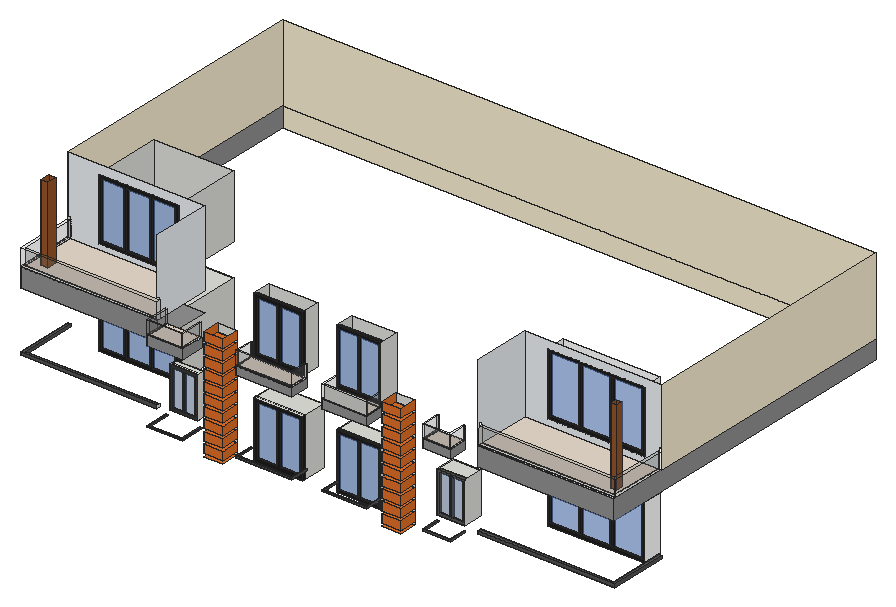
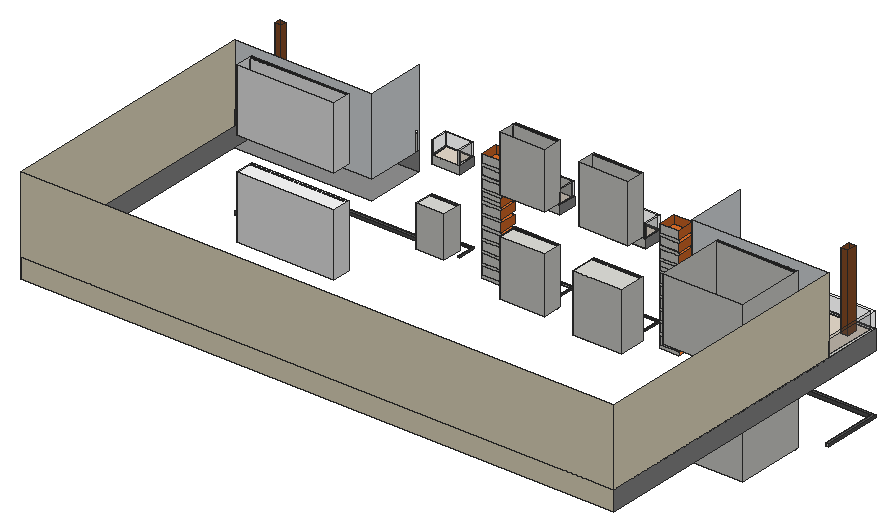
# SketchUp Ruby script. Lengths in inches.
U = 1.inch
M = Sketchup.active_model
def pt(a) = Geom::Point3d.new(a.map { |v| v * U })
def face(e, loops, mat)
  f = e.add_face(loops[0].map { |a| pt(a) })
  loops[1..].each { |l| e.add_face(l.map { |a| pt(a) }).erase! }
  f.material = f.back_material = mat if mat
  f
end
# faces: each face lists its corners as indices into pts; further lists are holes
def faces(e, pts, list, mat = nil) = list.each { |f| face(e, (f[0].is_a?(Array) ? f : [f]).map { |l| l.map { |i| pts[i] } }, mat) }
# xy, xz, yz: faces in a plane at the given z, y or x. An outline is a flat list of corners, or four numbers for a rectangle; further outlines are holes
def ring(l) = l.size == 4 ? [[l[0], l[1]], [l[2], l[1]], [l[2], l[3]], [l[0], l[3]]] : l.each_slice(2).to_a
def flat(e, list, mat, &to3) = list.each { |f| face(e, (f[0].is_a?(Array) ? f : [f]).map { |l| ring(l).map { |u, v| to3.(u, v) } }, mat) }
def xy(e, z, list, mat = nil) = flat(e, list, mat) { |x, y| [x, y, z] }
def xz(e, y, list, mat = nil) = flat(e, list, mat) { |x, z| [x, y, z] }
def yz(e, x, list, mat = nil) = flat(e, list, mat) { |y, z| [x, y, z] }
def lines(e, pts, list) = list.each { |a, b| e.add_line(pt(pts[a]), pt(pts[b])) }
# prism: a flat outline (further loops are holes) pulled along v
def prism(e, loops, v, mat = nil)
  f = face(e, loops, mat); d = Geom::Vector3d.new(v.map { |x| x * U })
  f.pushpull(f.normal.samedirection?(d) ? d.length : -d.length)
end
def box(e, o, s, mat = nil) = prism(e, [[o, [o[0] + s[0], o[1], o[2]], [o[0] + s[0], o[1] + s[1], o[2]], [o[0], o[1] + s[1], o[2]]]], [0, 0, s[2]], mat)
def at(x, y, z, deg = 0) = Geom::Transformation.translation(pt([x, y, z])) * Geom::Transformation.rotation(ORIGIN, Z_AXIS, deg.degrees)
def axes(o, x, y, z) = Geom::Transformation.new([*x, 0, *y, 0, *z, 0, *pt(o).to_a, 1])
def part(name) = M.definitions.add(name)
# library, detail: a bought-in or finely detailed component or shape, given as its bounding box
def library(name, o, s) = part(name).tap { |d| box(d.entities, o, s) }
def detail(e, o, s) = box(e.add_group.entities, o, s)
def put(e, d, t, mat = nil) = e.add_instance(d, t).tap { |i| i.material = mat if mat }
def group(e, t, mat = nil) = e.add_group.tap { |g| g.transformation = t; g.material = mat if mat }.entities
root = M.entities
M.materials.add("Generic").color = [146, 146, 146]
M.materials.add("Generic\#3").color = [226, 112, 41]
M.materials.add("Generic\#4").color = [237, 241, 244]
M.materials.add("Generic\#5").color = [249, 239, 211]
M.materials.add("Generic\#7").color = [232, 220, 205]
M.materials.add("[Color M00]").color = [255, 255, 255]
M.materials.add("[Color M06]").color = [86, 86, 86]
M.materials.add("[Color M07]").color = [58, 58, 58]
M.materials.add("[Color M08]").color = [30, 30, 30]
M.materials.add("[Translucent Glass Blue]").color = [98, 147, 234]
M.materials["[Translucent Glass Blue]"].alpha = 0.27
M.materials.add("[Translucent Glass Blue]1").color = [100, 149, 237]
M.materials["[Translucent Glass Blue]1"].alpha = 0.5
M.materials.add("[Translucent Glass Gray]").color = [119, 119, 119]
M.materials["[Translucent Glass Gray]"].alpha = 0.16
M.materials.add("[Wood Cherry Original]").color = [150, 85, 41]
M.materials.add("[Wood Cherry Original]1").color = [152, 86, 42]
c1 = part("Group\#10")
xy(c1.entities,0,[[0,0,98.1875,6]],"[Color M08]")
xy(c1.entities,5.79,[[5.79,0,46.2,3],[51.99,0,92.4,3]],"[Color M08]")
xy(c1.entities,117.02,[[5.79,0,46.2,3],[51.99,0,92.4,3]],"[Color M08]")
xy(c1.entities,122.8125,[[0,0,98.1875,6]],"[Color M08]")
xz(c1.entities,0,[[[0,0,98.1875,122.8125],[5.79,5.79,46.2,117.02],[51.99,5.79,92.4,117.02]]],"[Color M08]")
xz(c1.entities,3,[[5.79,5.79,46.2,117.02],[51.99,5.79,92.4,117.02]],"[Translucent Glass Blue]1")
xz(c1.entities,6,[[0,0,98.1875,122.8125]])
yz(c1.entities,0,[[0,0,6,122.8125]],"[Color M08]")
yz(c1.entities,5.79,[[0,5.79,3,117.02]],"[Color M08]")
yz(c1.entities,46.2,[[0,5.79,3,117.02]],"[Color M08]")
yz(c1.entities,51.99,[[0,5.79,3,117.02]],"[Color M08]")
yz(c1.entities,92.4,[[0,5.79,3,117.02]],"[Color M08]")
yz(c1.entities,98.1875,[[0,0,6,122.8125]],"[Color M08]")
c2 = part("Group\#11")
xy(c2.entities,0,[[0,0,175.8125,6]],"[Color M08]")
xy(c2.entities,7.33,[[7.33,0,56.16,3],[63.49,0,112.32,3],[119.65,0,168.48,3]],"[Color M08]")
xy(c2.entities,131.1,[[7.33,0,56.16,3],[63.49,0,112.32,3],[119.65,0,168.48,3]],"[Color M08]")
xy(c2.entities,138.4375,[[0,0,175.8125,6]],"[Color M08]")
xz(c2.entities,0,[[[0,0,175.8125,0,175.8125,131.1,168.48,131.1,168.48,7.33,119.65,7.33,119.65,131.1,175.8125,131.1,175.8125,138.4375,0,138.4375],[7.33,7.33,56.16,131.1],[63.49,7.33,112.32,131.1]]],"[Color M08]")
xz(c2.entities,3,[[7.33,7.33,56.16,131.1],[63.49,7.33,112.32,131.1],[119.65,7.33,168.48,131.1]],"[Translucent Glass Blue]1")
xz(c2.entities,6,[[0,0,175.8125,138.4375]])
yz(c2.entities,0,[[0,0,6,138.4375]],"[Color M08]")
yz(c2.entities,7.33,[[0,7.33,3,131.1]],"[Color M08]")
yz(c2.entities,56.16,[[0,7.33,3,131.1]],"[Color M08]")
yz(c2.entities,63.49,[[0,7.33,3,131.1]],"[Color M08]")
yz(c2.entities,112.32,[[0,7.33,3,131.1]],"[Color M08]")
yz(c2.entities,119.65,[[0,7.33,3,131.1]],"[Color M08]")
yz(c2.entities,168.48,[[0,7.33,3,131.1]],"[Color M08]")
yz(c2.entities,175.8125,[[0,0,6,138.4375]],"[Color M08]")
c3 = part("Group\#12")
xy(c3.entities,0,[[0,0,212.5625,7]],"[Color M08]")
xy(c3.entities,6.29,[[6.29,0,68.76,4],[75.05,0,137.52,4],[143.8,0,206.27,4]],"[Color M08]")
xy(c3.entities,131.21,[[6.29,0,68.76,4],[75.05,0,137.52,4],[143.8,0,206.27,4]],"[Color M08]")
xy(c3.entities,137.5,[[0,0,212.5625,7]],"[Color M08]")
xz(c3.entities,0,[[0,0,212.5625,6.29],[0,6.29,6.29,131.21],[68.76,6.29,75.05,131.21],[137.52,6.29,143.8,131.21],[206.27,6.29,212.5625,131.21],
  [0,131.21,212.5625,137.5]],"[Color M08]")
xz(c3.entities,4,[[6.29,6.29,68.76,131.21],[75.05,6.29,137.52,131.21],[143.8,6.29,206.27,131.21]],"[Translucent Glass Blue]1")
xz(c3.entities,7,[[0,0,212.5625,137.5]],"[Color M00]")
yz(c3.entities,0,[[0,0,7,137.5]],"[Color M08]")
yz(c3.entities,6.29,[[0,6.29,4,131.21]],"[Color M08]")
yz(c3.entities,68.76,[[0,6.29,4,131.21]],"[Color M08]")
yz(c3.entities,75.05,[[0,6.29,4,131.21]],"[Color M08]")
yz(c3.entities,137.52,[[0,6.29,4,131.21]],"[Color M08]")
yz(c3.entities,143.8,[[0,6.29,4,131.21]],"[Color M08]")
yz(c3.entities,206.27,[[0,6.29,4,131.21]],"[Color M08]")
yz(c3.entities,212.5625,[[0,0,7,137.5]],"[Color M08]")
c4 = part("Group\#1")
xy(c4.entities,0,[[0,0,60.75,6]],"[Color M07]")
xy(c4.entities,5.51,[[5.51,0,27.62,3],[33.13,0,55.24,3]],"[Color M07]")
xy(c4.entities,84.62,[[5.51,0,27.62,3],[33.13,0,55.24,3]])
xy(c4.entities,90.125,[[0,0,60.75,6]],"[Color M07]")
xz(c4.entities,0,[[[0,0,60.75,90.125],[5.51,5.51,27.62,84.62],[33.13,5.51,55.24,84.62]]],"[Color M07]")
xz(c4.entities,3,[[5.51,5.51,27.62,84.62],[33.13,5.51,55.24,84.62]],"[Translucent Glass Blue]")
xz(c4.entities,6,[[0,0,60.75,90.125]])
yz(c4.entities,0,[[0,0,6,90.125]],"[Color M07]")
yz(c4.entities,5.51,[[0,5.51,3,84.62]],"[Color M07]")
yz(c4.entities,27.62,[[0,5.51,3,84.62]],"[Color M07]")
yz(c4.entities,33.13,[[0,5.51,3,84.62]],"[Color M07]")
yz(c4.entities,55.24,[[0,5.51,3,84.62]],"[Color M07]")
yz(c4.entities,60.75,[[0,0,6,90.125]],"[Color M07]")
c5 = part("Group\#2")
xy(c5.entities,0,[[0,0,60.75,6]],"[Color M06]")
xy(c5.entities,4.875,[[4.875,0,27.9375,3],[32.8125,0,55.875,3]],"[Color M06]")
xy(c5.entities,85.25,[[4.875,0,27.9375,3],[32.8125,0,55.875,3]],"[Color M06]")
xy(c5.entities,90.125,[[0,0,60.75,6]],"[Color M06]")
xz(c5.entities,0,[[[0,0,60.75,90.125],[4.875,4.875,27.9375,85.25],[32.8125,4.875,55.875,85.25]]],"[Color M06]")
xz(c5.entities,3,[[4.875,4.875,27.9375,85.25],[32.8125,4.875,55.875,85.25]],"[Translucent Glass Blue]")
xz(c5.entities,6,[[0,0,60.75,90.125]])
yz(c5.entities,0,[[0,0,6,90.125]],"[Color M06]")
yz(c5.entities,4.875,[[0,4.875,3,85.25]],"[Color M06]")
yz(c5.entities,27.9375,[[0,4.875,3,85.25]],"[Color M06]")
yz(c5.entities,32.8125,[[0,4.875,3,85.25]],"[Color M06]")
yz(c5.entities,55.875,[[0,4.875,3,85.25]],"[Color M06]")
yz(c5.entities,60.75,[[0,0,6,90.125]],"[Color M06]")
xy(root,849.87,[[643.375,273.75,685.0625,313.625],[1034.5,273.75,1076.1875,313.625]],"Generic\#3")
xy(root,850.52,[[722.84,313.625,830.21,370.9375]])
xy(root,853.59,[[903.71,313.625,1001.9,356.375]])
xy(root,853.63,[[276.39,444.3125,452.2,595.9375]])
xy(root,856.37,[[643.375,273.75,685.0625,313.625],[1034.5,273.75,1076.1875,313.625]],"Generic\#3")
xy(root,856.82,[[1262.61,444.3125,1475.18,486.125]],"[Color M00]")
xy(root,873,[[529.46,261.625,529.46,313.625,532.46,313.625,532.46,264.625,604.09,264.625,604.09,313.625,607.09,313.625,607.09,261.625],[714.9,273.75,838.15,276.75],[903.71,273.75,906.71,313.625],[906.71,273.75,1001.9,276.75],[1125.09,273.75,1185.84,276.75],
  [714.9,276.75,717.9,313.625],[835.15,276.75,838.15,313.625],[998.9,276.75,1001.9,313.625],[1125.09,276.75,1128.09,313.625],[1182.84,276.75,1185.84,313.625]])
xy(root,874.37,[[643.375,273.75,685.0625,313.625],[1034.5,273.75,1076.1875,313.625]],"Generic\#3")
xy(root,875.75,[[529.46,261.625,607.09,261.625,607.09,313.625,604.09,313.625,604.09,264.625,532.46,264.625,532.46,313.625,529.46,313.625]],"[Color M06]")
xy(root,876,[[714.9,273.75,838.15,273.75,838.15,313.625,835.15,313.625,835.15,276.75,717.9,276.75,717.9,313.625,714.9,313.625],[903.71,273.75,1001.9,273.75,1001.9,313.625,998.9,313.625,998.9,276.75,906.71,276.75,906.71,313.625,903.71,313.625],[1125.09,273.75,1185.84,273.75,1185.84,313.625,1182.84,313.625,1182.84,276.75,1128.09,276.75,1128.09,313.625,1125.09,313.625]],"[Color M06]")
xy(root,879,[[209.5,313.625,209.5,444.3125,216.5,444.3125,216.5,320.625,509.5,320.625,509.5,313.625],[1213,316.0625,1213,323.0625,1506,323.0625,1506,444.3125,1513,444.3125,1513,316.0625]])
xy(root,880.87,[[643.375,273.75,685.0625,313.625],[1034.5,273.75,1076.1875,313.625]],"Generic\#3")
xy(root,885.4375,[[1213,316.0625,1513,316.0625,1513,444.3125,1506,444.3125,1506,323.0625,1213,323.0625]],"[Color M06]")
xy(root,886,[[209.5,313.625,509.5,313.625,509.5,320.625,216.5,320.625,216.5,444.3125,209.5,444.3125]],"[Color M06]")
xy(root,886.27,[[537.9,313.625,598.65,331.25]])
xy(root,887.24,[[1125.09,313.625,1185.84,356.375]])
xy(root,898.87,[[643.375,273.75,685.0625,313.625],[1034.5,273.75,1076.1875,313.625]],"Generic\#3")
xy(root,905.37,[[643.375,273.75,685.0625,313.625],[1034.5,273.75,1076.1875,313.625]],"Generic\#3")
xy(root,923.37,[[643.375,273.75,685.0625,313.625],[1034.5,273.75,1076.1875,313.625]],"Generic\#3")
xy(root,929.87,[[643.375,273.75,685.0625,313.625],[1034.5,273.75,1076.1875,313.625]],"Generic\#3")
xy(root,947.87,[[643.375,273.75,685.0625,313.625],[1034.5,273.75,1076.1875,313.625]],"Generic\#3")
xy(root,954.37,[[643.375,273.75,685.0625,313.625],[1034.5,273.75,1076.1875,313.625]],"Generic\#3")
xy(root,972.37,[[643.375,273.75,685.0625,313.625],[1034.5,273.75,1076.1875,313.625]],"Generic\#3")
xy(root,976.4,[[537.9,313.625,598.65,331.25],[722.84,313.625,830.21,370.9375],[903.71,313.625,1001.9,356.375]])
xy(root,977.36,[[1125.09,313.625,1185.84,356.375]])
xy(root,978.87,[[643.375,273.75,685.0625,313.625],[1034.5,273.75,1076.1875,313.625]],"Generic\#3")
xy(root,992.07,[[276.39,444.3125,452.2,595.9375]])
xy(root,994.32,[[1262.61,444.3125,1475.18,486.125]],"[Color M00]")
xy(root,996.87,[[643.375,273.75,685.0625,313.625],[1034.5,273.75,1076.1875,313.625]],"Generic\#3")
xy(root,1003.37,[[643.375,273.75,685.0625,313.625],[1034.5,273.75,1076.1875,313.625]],"Generic\#3")
xy(root,1011,[[[209.5,313.625,509.5,444.3125],[234.12,340.02,249.74,361.77]],[[1213,313.625,1513,444.3125],[1483.76,340.63,1497.19,353.98]]],"Generic")
xy(root,1021.37,[[643.375,273.75,685.0625,313.625],[1034.5,273.75,1076.1875,313.625]],"Generic\#3")
xy(root,1027.87,[[643.375,273.75,685.0625,313.625],[1034.5,273.75,1076.1875,313.625]],"Generic\#3")
xy(root,1032.375,[[529.46,261.625,607.09,313.625]],"Generic")
xy(root,1035.3125,[[714.9,273.75,838.15,313.625],[903.71,273.75,1001.9,313.625],[1125.09,273.75,1185.84,313.625]],"Generic")
xy(root,1045.87,[[643.375,273.75,685.0625,313.625],[1034.5,273.75,1076.1875,313.625]],"Generic\#3")
xy(root,1052.37,[[643.375,273.75,685.0625,313.625],[1034.5,273.75,1076.1875,313.625]],"Generic\#3")
xy(root,1053.75,[[529.46,261.625,529.46,313.625,532.46,313.625,532.46,264.625,604.09,264.625,604.09,313.625,607.09,313.625,607.09,261.625],[714.9,273.75,838.15,276.75],[903.71,273.75,1001.9,276.75],[1125.09,273.75,1185.84,276.75],[714.9,276.75,717.9,313.625],
  [835.15,276.75,838.15,313.625],[903.71,276.75,906.71,313.625],[998.9,276.75,1001.9,313.625],[1125.09,276.75,1128.09,313.625],[1182.84,276.75,1185.84,313.625],
  [209.5,313.625,509.5,320.625],[1213,313.625,1513,318.25],[1213,318.25,1213,325.0625,1506,325.0625,1506,444.3125,1513,444.3125,1513,318.25],[209.5,320.625,216.5,444.3125],[234.12,340.02,249.74,361.77],
  [1483.76,340.63,1497.19,353.98]])
xy(root,1053.75,[[532.46,264.625,604.09,313.625],[717.9,276.75,835.15,313.625],[906.71,276.75,998.9,313.625],[1128.09,276.75,1182.84,313.625],[[216.5,320.625,509.5,444.3125],[234.12,340.02,249.74,361.77]],
  [[1213,325.0625,1506,444.3125],[1483.76,340.63,1497.19,353.98]]],"Generic\#7")
xy(root,1056.17,[[722.84,313.625,830.21,354]])
xy(root,1059.34,[[903.71,313.625,1001.9,356.375]])
xy(root,1063.63,[[276.39,444.3125,452.2,595.9375]])
xy(root,1067.01,[[1262.61,444.3125,1475.18,486.125]],"[Color M00]")
xy(root,1070.37,[[643.375,273.75,685.0625,313.625],[1034.5,273.75,1076.1875,313.625]],"Generic\#3")
xy(root,1076.87,[[643.375,273.75,685.0625,313.625],[1034.5,273.75,1076.1875,313.625]],"Generic\#3")
xz(root,261.625,[[529.46,1032.375,607.09,1053.75]],"Generic")
xz(root,261.625,[[529.46,873,607.09,875.75]],"[Color M06]")
xz(root,261.625,[[529.46,1053.75,607.09,1083.75]],"[Translucent Glass Gray]")
xz(root,264.625,[[532.46,873,604.09,875.75]])
xz(root,264.625,[[532.46,1053.75,604.09,1083.75]],"[Translucent Glass Gray]")
xz(root,273.75,[[714.9,1035.3125,838.15,1053.75],[903.71,1035.3125,1001.9,1053.75],[1125.09,1035.3125,1185.84,1053.75]],"Generic")
xz(root,273.75,[[643.375,856.37,685.0625,874.37],[1034.5,856.37,1076.1875,874.37],[643.375,880.87,685.0625,898.87],[1034.5,880.87,1076.1875,898.87],[643.375,905.37,685.0625,923.37],
  [1034.5,905.37,1076.1875,923.37],[643.375,929.87,685.0625,947.87],[1034.5,929.87,1076.1875,947.87],[643.375,954.37,685.0625,972.37],[1034.5,954.37,1076.1875,972.37],
  [643.375,978.87,685.0625,996.87],[1034.5,978.87,1076.1875,996.87],[643.375,1003.37,685.0625,1021.37],[1034.5,1003.37,1076.1875,1021.37],[643.375,1027.87,685.0625,1045.87],
  [1034.5,1027.87,1076.1875,1045.87],[643.375,1052.37,685.0625,1070.37],[1034.5,1052.37,1076.1875,1070.37],[643.375,1076.87,685.0625,1094.87],[1034.5,1076.87,1076.1875,1094.87]],"Generic\#3")
xz(root,273.75,[[714.9,873,838.15,876],[903.71,873,1001.9,876],[1125.09,873,1185.84,876]],"[Color M06]")
xz(root,273.75,[[714.9,1053.75,838.15,1083.75],[903.71,1053.75,1001.9,1083.75],[1125.09,1053.75,1185.84,1083.75]],"[Translucent Glass Gray]")
xz(root,276.75,[[717.9,873,835.15,876],[906.71,873,998.9,876],[1128.09,873,1182.84,876],[906.71,1053.75,998.9,1083.75]])
xz(root,276.75,[[717.9,1053.75,835.15,1083.75],[1128.09,1053.75,1182.84,1083.75]],"[Translucent Glass Gray]")
xz(root,313.625,[[643.375,849.87,685.0625,856.37],[1034.5,849.87,1076.1875,856.37],[903.71,853.59,906.71,873],[998.9,853.59,1001.9,873],[643.375,856.37,685.0625,874.37],
  [1034.5,856.37,1076.1875,874.37],[714.9,873,717.9,876],[835.15,873,838.15,876],[903.71,873,906.71,876],[998.9,873,1001.9,876],
  [1125.09,873,1128.09,876],[1182.84,873,1185.84,876],[643.375,874.37,685.0625,880.87],[1034.5,874.37,1076.1875,880.87],[643.375,880.87,685.0625,898.87],
  [1034.5,880.87,1076.1875,898.87],[643.375,898.87,685.0625,905.37],[1034.5,898.87,1076.1875,905.37],[643.375,905.37,685.0625,923.37],[1034.5,905.37,1076.1875,923.37],
  [643.375,923.37,685.0625,929.87],[1034.5,923.37,1076.1875,929.87],[643.375,929.87,685.0625,947.87],[1034.5,929.87,1076.1875,947.87],[643.375,947.87,685.0625,954.37],
  [1034.5,947.87,1076.1875,954.37],[643.375,954.37,685.0625,972.37],[1034.5,954.37,1076.1875,972.37],[643.375,972.37,685.0625,978.87],[1034.5,972.37,1076.1875,978.87],
  [643.375,978.87,685.0625,996.87],[1034.5,978.87,1076.1875,996.87],[643.375,996.87,685.0625,1003.37],[1034.5,996.87,1076.1875,1003.37],[643.375,1003.37,685.0625,1011],
  [1034.5,1003.37,1076.1875,1011],[643.375,1011,685.0625,1021.37],[1034.5,1011,1076.1875,1021.37],[643.375,1021.37,685.0625,1027.87],[1034.5,1021.37,1076.1875,1027.87],
  [643.375,1027.87,685.0625,1045.87],[1034.5,1027.87,1076.1875,1045.87],[529.46,1032.375,607.09,1053.75],[714.9,1035.3125,838.15,1053.75],[903.71,1035.3125,1001.9,1053.75],
  [1125.09,1035.3125,1185.84,1053.75],[643.375,1045.87,685.0625,1052.37],[1034.5,1045.87,1076.1875,1052.37],[643.375,1052.37,685.0625,1053.75],[1034.5,1052.37,1076.1875,1053.75],
  [643.375,1053.75,685.0625,1070.37],[714.9,1053.75,717.9,1083.75],[835.15,1053.75,838.15,1083.75],[903.71,1053.75,906.71,1059.34],[906.71,1053.75,998.9,1059.34],
  [998.9,1053.75,1001.9,1059.34],[1034.5,1053.75,1076.1875,1070.37],[1125.09,1053.75,1128.09,1083.75],[1182.84,1053.75,1185.84,1083.75],[903.71,1059.34,906.71,1083.75],
  [998.9,1059.34,1001.9,1083.75],[643.375,1070.37,685.0625,1076.87],[1034.5,1070.37,1076.1875,1076.87],[643.375,1076.87,685.0625,1094.87],[1034.5,1076.87,1076.1875,1094.87]])
xz(root,313.625,[[209.5,1011,509.5,1053.75],[1213,1011,1513,1053.75]],"Generic")
xz(root,313.625,[[209.5,879,509.5,886]],"[Color M06]")
xz(root,313.625,[[209.5,1053.75,509.5,1089.75]],"[Translucent Glass Gray]")
xz(root,316.0625,[[1213,879,1513,885.4375]],"[Color M06]")
xz(root,318.25,[[1213,1053.75,1513,1089.75]],"[Translucent Glass Gray]")
xz(root,320.625,[[216.5,879,509.5,886]],"[Color M06]")
xz(root,320.625,[[216.5,1053.75,509.5,1089.75]],"[Translucent Glass Gray]")
xz(root,323.0625,[[1213,879,1506,885.4375]],"[Color M06]")
xz(root,325.0625,[[1213,1053.75,1506,1089.75]],"[Translucent Glass Gray]")
xz(root,331.25,[[537.9,886.27,598.65,976.4]])
xz(root,340.02,[[234.12,1053.75,249.74,1221.75]],"[Wood Cherry Original]1")
xz(root,340.63,[[1483.76,1053.75,1497.19,1221.75]],"[Wood Cherry Original]")
xz(root,353.98,[[1483.76,1053.75,1497.19,1221.75]],"[Wood Cherry Original]")
xz(root,354,[[722.84,1056.17,830.21,1182.05]])
xz(root,356.375,[[903.71,853.59,1001.9,976.4],[1125.09,887.24,1185.84,977.36],[903.71,1059.34,1001.9,1182.15]])
xz(root,361.77,[[234.12,1053.75,249.74,1221.75]],"[Wood Cherry Original]1")
xz(root,370.9375,[[722.84,850.52,830.21,976.4]])
xz(root,444.3125,[[209.5,879,216.5,886],[209.5,1053.75,216.5,1089.75]])
xz(root,444.3125,[[[216.5,1053.75,509.5,1053.75,509.5,1221.75,209.5,1221.75,209.5,1096.75,216.5,1096.75],[276.39,1063.63,452.2,1202.07]],[[1213,1053.75,1506,1053.75,1506,1096.1875,1513,1096.1875,1513,1221.75,1213,1221.75],[1262.61,1067.01,1475.18,1204.51]]],"Generic\#4")
xz(root,486.125,[[1262.61,856.82,1475.18,994.32],[1262.61,1067.01,1475.18,1204.51]],"[Color M00]")
xz(root,595.9375,[[276.39,853.63,452.2,992.07],[276.39,1063.63,452.2,1202.07]])
xz(root,1033.625,[[209.5,1011,1513,1053.75],[209.5,1053.75,1513,1221.75]],"Generic\#5")
yz(root,209.5,[[313.625,1011,1033.625,1053.75]],"Generic")
yz(root,209.5,[[444.3125,1053.75,1033.625,1221.75]],"Generic\#5")
yz(root,209.5,[[313.625,879,444.3125,886]],"[Color M06]")
yz(root,209.5,[[313.625,1053.75,444.3125,1089.75]],"[Translucent Glass Gray]")
yz(root,216.5,[[320.625,879,444.3125,886]],"[Color M06]")
yz(root,216.5,[[320.625,1053.75,444.3125,1089.75]],"[Translucent Glass Gray]")
yz(root,234.12,[[340.02,1053.75,361.77,1221.75]],"[Wood Cherry Original]1")
yz(root,249.74,[[340.02,1053.75,361.77,1221.75]],"[Wood Cherry Original]1")
yz(root,276.39,[[444.3125,853.63,595.9375,992.07],[444.3125,1063.63,595.9375,1202.07]])
yz(root,452.2,[[444.3125,853.63,595.9375,992.07],[444.3125,1063.63,595.9375,1202.07]])
yz(root,509.5,[[313.625,879,320.625,886],[313.625,1053.75,320.625,1089.75]])
yz(root,509.5,[[320.625,1053.75,320.625,1096.75,313.625,1096.75,313.625,1221.75,444.3125,1221.75,444.3125,1053.75]],"Generic\#4")
yz(root,529.46,[[261.625,1032.375,313.625,1053.75]],"Generic")
yz(root,529.46,[[261.625,873,313.625,875.75]],"[Color M06]")
yz(root,529.46,[[261.625,1053.75,313.625,1083.75]],"[Translucent Glass Gray]")
yz(root,532.46,[[264.625,873,313.625,875.75]],"[Color M06]")
yz(root,532.46,[[264.625,1053.75,313.625,1083.75]],"[Translucent Glass Gray]")
yz(root,537.9,[[313.625,886.27,331.25,976.4]])
yz(root,598.65,[[313.625,886.27,331.25,976.4]])
yz(root,604.09,[[264.625,873,313.625,875.75]],"[Color M06]")
yz(root,604.09,[[264.625,1053.75,313.625,1083.75]],"[Translucent Glass Gray]")
yz(root,607.09,[[261.625,1032.375,313.625,1053.75]],"Generic")
yz(root,607.09,[[261.625,873,313.625,875.75]],"[Color M06]")
yz(root,607.09,[[261.625,1053.75,313.625,1083.75]],"[Translucent Glass Gray]")
yz(root,643.375,[[273.75,856.37,313.625,874.37],[273.75,880.87,313.625,898.87],[273.75,905.37,313.625,923.37],[273.75,929.87,313.625,947.87],[273.75,954.37,313.625,972.37],
  [273.75,978.87,313.625,996.87],[273.75,1003.37,313.625,1021.37],[273.75,1027.87,313.625,1045.87],[273.75,1052.37,313.625,1070.37],[273.75,1076.87,313.625,1094.87]],"Generic\#3")
yz(root,685.0625,[[273.75,856.37,313.625,874.37],[273.75,880.87,313.625,898.87],[273.75,905.37,313.625,923.37],[273.75,929.87,313.625,947.87],[273.75,954.37,313.625,972.37],
  [273.75,978.87,313.625,996.87],[273.75,1003.37,313.625,1021.37],[273.75,1027.87,313.625,1045.87],[273.75,1052.37,313.625,1070.37],[273.75,1076.87,313.625,1094.87]],"Generic\#3")
yz(root,714.9,[[273.75,1035.3125,313.625,1053.75]],"Generic")
yz(root,714.9,[[273.75,873,313.625,876]],"[Color M06]")
yz(root,714.9,[[273.75,1053.75,313.625,1083.75]],"[Translucent Glass Gray]")
yz(root,717.9,[[276.75,873,313.625,876]],"[Color M06]")
yz(root,717.9,[[276.75,1053.75,313.625,1083.75]],"[Translucent Glass Gray]")
yz(root,722.84,[[313.625,850.52,370.9375,976.4],[313.625,1056.17,354,1182.05]])
yz(root,830.21,[[313.625,850.52,370.9375,976.4],[313.625,1056.17,354,1182.05]])
yz(root,835.15,[[276.75,873,313.625,876]],"[Color M06]")
yz(root,835.15,[[276.75,1053.75,313.625,1083.75]],"[Translucent Glass Gray]")
yz(root,838.15,[[273.75,1035.3125,313.625,1053.75]],"Generic")
yz(root,838.15,[[273.75,873,313.625,876]],"[Color M06]")
yz(root,838.15,[[273.75,1053.75,313.625,1083.75]],"[Translucent Glass Gray]")
yz(root,903.71,[[313.625,853.59,356.375,976.4],[313.625,1059.34,356.375,1182.15]])
yz(root,903.71,[[273.75,1035.3125,313.625,1053.75]],"Generic")
yz(root,903.71,[[273.75,873,313.625,876]],"[Color M06]")
yz(root,903.71,[[273.75,1053.75,313.625,1083.75]],"[Translucent Glass Gray]")
yz(root,906.71,[[276.75,873,313.625,876]],"[Color M06]")
yz(root,906.71,[[276.75,1053.75,313.625,1083.75]],"[Translucent Glass Gray]")
yz(root,998.9,[[276.75,873,313.625,876]],"[Color M06]")
yz(root,998.9,[[276.75,1053.75,313.625,1083.75]],"[Translucent Glass Gray]")
yz(root,1001.9,[[313.625,853.59,356.375,976.4],[313.625,1059.34,356.375,1182.15]])
yz(root,1001.9,[[273.75,1035.3125,313.625,1053.75]],"Generic")
yz(root,1001.9,[[273.75,873,313.625,876]],"[Color M06]")
yz(root,1001.9,[[273.75,1053.75,313.625,1083.75]],"[Translucent Glass Gray]")
yz(root,1034.5,[[273.75,856.37,313.625,874.37],[273.75,880.87,313.625,898.87],[273.75,905.37,313.625,923.37],[273.75,929.87,313.625,947.87],[273.75,954.37,313.625,972.37],
  [273.75,978.87,313.625,996.87],[273.75,1003.37,313.625,1021.37],[273.75,1027.87,313.625,1045.87],[273.75,1052.37,313.625,1070.37],[273.75,1076.87,313.625,1094.87]],"Generic\#3")
yz(root,1076.1875,[[273.75,856.37,313.625,874.37],[273.75,880.87,313.625,898.87],[273.75,905.37,313.625,923.37],[273.75,929.87,313.625,947.87],[273.75,954.37,313.625,972.37],
  [273.75,978.87,313.625,996.87],[273.75,1003.37,313.625,1021.37],[273.75,1027.87,313.625,1045.87],[273.75,1052.37,313.625,1070.37],[273.75,1076.87,313.625,1094.87]],"Generic\#3")
yz(root,1125.09,[[313.625,887.24,356.375,977.36]])
yz(root,1125.09,[[273.75,1035.3125,313.625,1053.75]],"Generic")
yz(root,1125.09,[[273.75,873,313.625,876]],"[Color M06]")
yz(root,1125.09,[[273.75,1053.75,313.625,1083.75]],"[Translucent Glass Gray]")
yz(root,1128.09,[[276.75,873,313.625,876]],"[Color M06]")
yz(root,1128.09,[[276.75,1053.75,313.625,1083.75]],"[Translucent Glass Gray]")
yz(root,1182.84,[[276.75,873,313.625,876]],"[Color M06]")
yz(root,1182.84,[[276.75,1053.75,313.625,1083.75]],"[Translucent Glass Gray]")
yz(root,1185.84,[[313.625,887.24,356.375,977.36]])
yz(root,1185.84,[[273.75,1035.3125,313.625,1053.75]],"Generic")
yz(root,1185.84,[[273.75,873,313.625,876]],"[Color M06]")
yz(root,1185.84,[[273.75,1053.75,313.625,1083.75]],"[Translucent Glass Gray]")
yz(root,1213,[[316.0625,879,323.0625,885.4375],[318.25,1053.75,325.0625,1089.75]])
yz(root,1213,[[313.625,1053.75,318.25,1053.75,318.25,1096.1875,325.0625,1096.1875,325.0625,1053.75,444.3125,1053.75,444.3125,1221.75,313.625,1221.75]],"Generic\#4")
yz(root,1262.61,[[444.3125,856.82,486.125,994.32],[444.3125,1067.01,486.125,1204.51]],"[Color M00]")
yz(root,1475.18,[[444.3125,856.82,486.125,994.32],[444.3125,1067.01,486.125,1204.51]],"[Color M00]")
yz(root,1483.76,[[340.63,1053.75,353.98,1221.75]],"[Wood Cherry Original]")
yz(root,1497.19,[[340.63,1053.75,353.98,1221.75]],"[Wood Cherry Original]")
yz(root,1506,[[323.0625,879,444.3125,885.4375]],"[Color M06]")
yz(root,1506,[[325.0625,1053.75,444.3125,1089.75]],"[Translucent Glass Gray]")
yz(root,1513,[[313.625,1011,1033.625,1053.75]],"Generic")
yz(root,1513,[[444.3125,1053.75,1033.625,1221.75]],"Generic\#5")
yz(root,1513,[[316.0625,879,444.3125,885.4375]],"[Color M06]")
yz(root,1513,[[318.25,1053.75,444.3125,1089.75]],"[Translucent Glass Gray]")
g1 = group(root,at(722.84,313.625,850.52))
xy(g1,0,[[0,0,107.375,6]],"[Color M08]")
xy(g1,7.85,[[7.85,0,49.76,3],[57.61,0,99.52,3]],"[Color M08]")
xy(g1,118.02,[[7.85,0,49.76,3],[57.61,0,99.52,3]],"[Color M08]")
xy(g1,125.875,[[0,0,107.375,6]],"[Color M08]")
xz(g1,0,[[[0,0,107.375,125.875],[57.61,7.85,99.52,118.02],[7.85,7.85,49.76,118.02]]],"[Color M08]")
xz(g1,3,[[7.85,7.85,49.76,118.02],[57.61,7.85,99.52,118.02]],"[Translucent Glass Blue]1")
xz(g1,6,[[0,0,107.375,125.875]])
yz(g1,0,[[0,0,6,125.875]],"[Color M08]")
yz(g1,7.85,[[0,7.85,3,118.02]],"[Color M08]")
yz(g1,49.76,[[0,7.85,3,118.02]],"[Color M08]")
yz(g1,57.61,[[0,7.85,3,118.02]],"[Color M08]")
yz(g1,99.52,[[0,7.85,3,118.02]],"[Color M08]")
yz(g1,107.375,[[0,0,6,125.875]],"[Color M08]")
put(root,c1,at(903.71,313.625,853.59))
put(root,c2,at(276.39,444.3125,853.63))
put(root,c3,at(1262.61,444.3125,856.82))
put(root,c4,at(537.9,313.625,886.27))
put(root,c5,at(1125.09,313.625,887.24))
g2 = group(root,at(722.84,313.625,1056.17))
xy(g2,0,[[0,0,107.375,6]],"[Color M08]")
xy(g2,7.89,[[7.89,0,49.74,3],[57.63,0,99.48,3]],"[Color M08]")
xy(g2,117.98,[[7.89,0,49.74,3],[57.63,0,99.48,3]],"[Color M08]")
xy(g2,125.875,[[0,0,107.375,6]],"[Color M08]")
xz(g2,0,[[[0,0,107.375,125.875],[57.63,7.89,99.48,117.98],[7.89,7.89,49.74,117.98]]],"[Color M08]")
xz(g2,3,[[7.89,7.89,49.74,117.98],[57.63,7.89,99.48,117.98]],"[Translucent Glass Blue]1")
xz(g2,6,[[0,0,107.375,125.875]])
yz(g2,0,[[0,0,6,125.875]],"[Color M08]")
yz(g2,7.89,[[0,7.89,3,117.98]],"[Color M08]")
yz(g2,49.74,[[0,7.89,3,117.98]],"[Color M08]")
yz(g2,57.63,[[0,7.89,3,117.98]],"[Color M08]")
yz(g2,99.48,[[0,7.89,3,117.98]],"[Color M08]")
yz(g2,107.375,[[0,0,6,125.875]],"[Color M08]")
put(root,c1,at(903.71,313.625,1059.34))
put(root,c2,at(276.39,444.3125,1063.63))
put(root,c3,at(1262.61,444.3125,1067.01))
